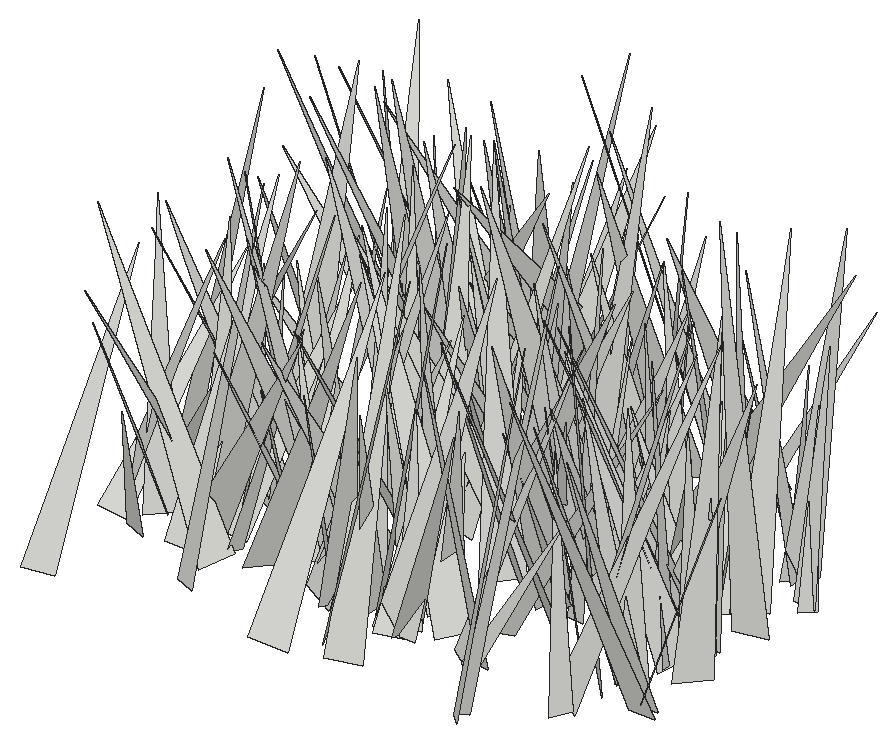
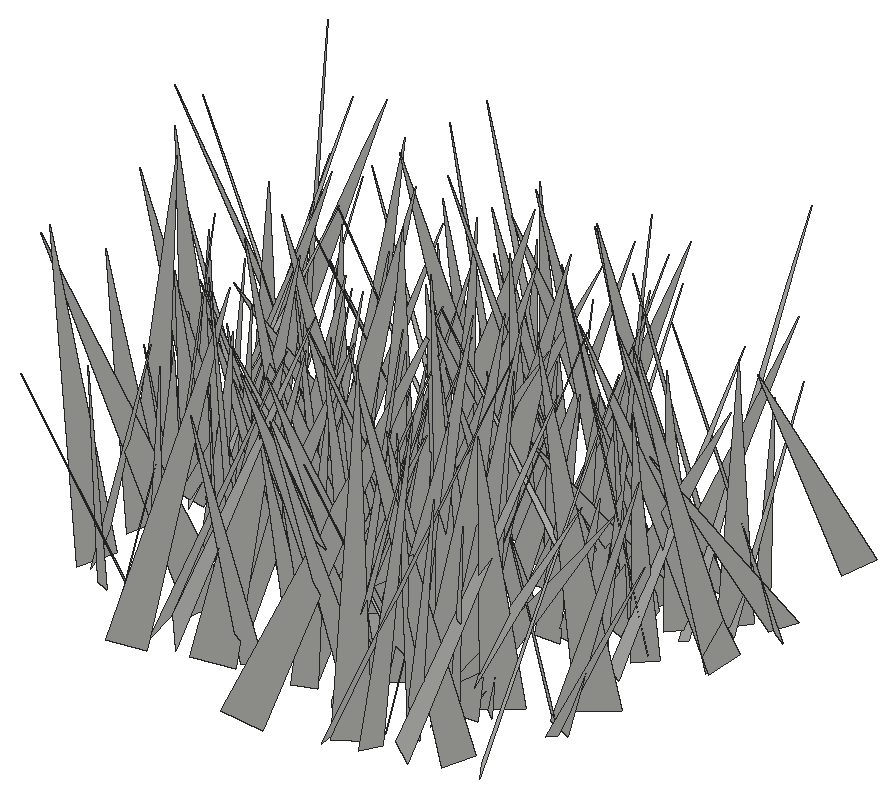
# SketchUp Ruby script. Lengths in inches.
U = 1.inch
M = Sketchup.active_model
def pt(a) = Geom::Point3d.new(a.map { |v| v * U })
def face(e, loops, mat)
  f = e.add_face(loops[0].map { |a| pt(a) })
  loops[1..].each { |l| e.add_face(l.map { |a| pt(a) }).erase! }
  f.material = f.back_material = mat if mat
  f
end
# faces: each face lists its corners as indices into pts; further lists are holes
def faces(e, pts, list, mat = nil) = list.each { |f| face(e, (f[0].is_a?(Array) ? f : [f]).map { |l| l.map { |i| pts[i] } }, mat) }
# xy, xz, yz: faces in a plane at the given z, y or x. An outline is a flat list of corners, or four numbers for a rectangle; further outlines are holes
def ring(l) = l.size == 4 ? [[l[0], l[1]], [l[2], l[1]], [l[2], l[3]], [l[0], l[3]]] : l.each_slice(2).to_a
def flat(e, list, mat, &to3) = list.each { |f| face(e, (f[0].is_a?(Array) ? f : [f]).map { |l| ring(l).map { |u, v| to3.(u, v) } }, mat) }
def xy(e, z, list, mat = nil) = flat(e, list, mat) { |x, y| [x, y, z] }
def xz(e, y, list, mat = nil) = flat(e, list, mat) { |x, z| [x, y, z] }
def yz(e, x, list, mat = nil) = flat(e, list, mat) { |y, z| [x, y, z] }
def lines(e, pts, list) = list.each { |a, b| e.add_line(pt(pts[a]), pt(pts[b])) }
# prism: a flat outline (further loops are holes) pulled along v
def prism(e, loops, v, mat = nil)
  f = face(e, loops, mat); d = Geom::Vector3d.new(v.map { |x| x * U })
  f.pushpull(f.normal.samedirection?(d) ? d.length : -d.length)
end
def box(e, o, s, mat = nil) = prism(e, [[o, [o[0] + s[0], o[1], o[2]], [o[0] + s[0], o[1] + s[1], o[2]], [o[0], o[1] + s[1], o[2]]]], [0, 0, s[2]], mat)
def at(x, y, z, deg = 0) = Geom::Transformation.translation(pt([x, y, z])) * Geom::Transformation.rotation(ORIGIN, Z_AXIS, deg.degrees)
def axes(o, x, y, z) = Geom::Transformation.new([*x, 0, *y, 0, *z, 0, *pt(o).to_a, 1])
def part(name) = M.definitions.add(name)
# library, detail: a bought-in or finely detailed component or shape, given as its bounding box
def library(name, o, s) = part(name).tap { |d| box(d.entities, o, s) }
def detail(e, o, s) = box(e.add_group.entities, o, s)
def put(e, d, t, mat = nil) = e.add_instance(d, t).tap { |i| i.material = mat if mat }
def group(e, t, mat = nil) = e.add_group.tap { |g| g.transformation = t; g.material = mat if mat }.entities
root = M.entities
c1 = part("fur_instance\#9")
p = [[0.8125,0,1.79],[0.67,-0.02,1.48],[0,-0.11,0],[0,0.11,0]]
faces(c1.entities,p,[[0,1,2,3]])
put(root,c1,axes([528.73,42.07,-21.86],[-0.43336,-3.79274,0.22877],[-3.61563,0.48241,1.14868],[1.16807,0.08612,3.64049]))
put(root,c1,axes([527.9,37.6,-21.86],[-4.59878,4.14257,0.47856],[3.69105,4.37512,-2.40275],[1.94062,1.49539,5.70408]))
put(root,c1,axes([538.61,40.67,-21.86],[7.04246,3.4796,1.7186],[3.70112,-7.09298,-0.80545],[-1.16744,-1.49647,7.81378]))
put(root,c1,axes([546.14,38.49,-21.86],[4.5947,4.98178,1.41698],[4.55399,-4.78808,2.06705],[-2.46722,0.43974,6.4542]))
put(root,c1,axes([529.47,45.59,-21.86],[-5.00279,-6.48805,0.18943],[-5.66686,4.48249,3.86684],[3.16501,-2.22958,7.22289]))
put(root,c1,axes([537.7,42.4,-21.86],[5.23742,-3.794,0.7561],[-3.79638,-5.28528,-0.22367],[-0.74406,0.26094,6.46336]))
put(root,c1,axes([537.62,38.52,-21.86],[-1.59566,7.05244,0.57454],[6.94745,1.67322,-1.24356],[1.34162,-0.27674,7.12297]))
put(root,c1,axes([551.11,42.86,-21.86],[-1.75901,-6.72397,0.92553],[-6.70142,1.56883,-1.33876],[-1.07676,1.22044,6.82009]))
put(root,c1,axes([540.875,42.35,-21.86],[5.31861,-1.95589,0.12332],[-1.94358,-5.30997,-0.39374],[-0.25139,-0.32717,5.65315]))
put(root,c1,axes([539,42.79,-21.86],[4.83805,-1.95602,0.87332],[-1.75837,-4.85831,-1.14034],[-1.22345,-0.75248,5.09238]))
put(root,c1,axes([544.34,41.36,-21.86],[2.38056,3.51502,0.37387],[3.33138,-2.08023,-1.65431],[1.18197,-1.21634,3.90969]))
put(root,c1,axes([530.85,43.33,-21.86],[2.77166,-6.45652,0.14972],[-5.9267,-2.47813,2.8503],[2.56578,1.25036,6.42219]))
put(root,c1,axes([548.87,41.07,-21.86],[-4.5869,1.43943,1.05541],[1.33614,4.69877,-0.60151],[1.18347,0.27406,4.76967]))
put(root,c1,axes([537.01,42.99,-21.86],[3.60771,1.96245,2.32029],[2.67745,-3.75626,-0.98607],[-1.43745,-2.07119,3.98679]))
put(root,c1,axes([550.94,43.3125,-21.86],[-0.82643,-5.48525,0.94931],[-5.54864,0.73423,-0.58792],[-0.44918,1.02229,5.51591]))
put(root,c1,axes([532.42,42.1,-21.86],[-6.66331,2.16551,0.21128],[2.17487,6.60915,0.85019],[-0.06344,-0.87375,6.95459]))
put(root,c1,axes([548.43,43.8,-21.86],[-5.2101,-5.93708,2.74108],[-5.84341,5.80017,1.45611],[2.93548,1.00834,7.76362]))
put(root,c1,axes([528.45,44.15,-21.86],[-3.04266,-3.74721,0.50143],[-3.60797,3.07034,1.05183],[1.12942,-0.28668,4.71094]))
put(root,c1,axes([534.29,45.22,-21.86],[-3.9218,-4.42687,0.35438],[-4.07666,3.77609,2.05553],[1.7617,-1.11678,5.54549]))
put(root,c1,axes([540.45,39.26,-21.86],[0.0768,8.17284,0.16546],[8.06568,-0.10268,1.32775],[-1.3295,-0.15078,8.06464]))
put(root,c1,axes([533.91,42.9,-21.86],[6.48225,-3.39085,0.68777],[-3.4557,-6.41712,0.9323],[-0.17042,1.14593,7.25591]))
put(root,c1,axes([544.57,42.02,-21.86],[-3.42492,-4.02626,1.68032],[-4.34426,2.9504,-1.78518],[-0.40205,2.41841,4.97534]))
put(root,c1,axes([540.84,42.4375,-21.86],[-2.37433,3.47563,1.70417],[3.72029,2.6012,-0.12184],[1.06942,-1.33243,4.20745]))
put(root,c1,axes([532.57,40.1,-21.86],[3.83849,6.3713,1.10198],[6.13828,-3.99344,1.70758],[-2.03209,-0.02789,7.23959]))
put(root,c1,axes([536.54,42.74,-21.86],[1.01992,4.1189,1.46608],[4.23417,-0.55549,-1.38501],[1.0893,-1.69737,4.0109]))
put(root,c1,axes([536.79,46.07,-21.86],[-6.04066,-0.63869,2.51357],[0.73038,5.69455,3.20222],[2.48847,-3.22176,5.16172]))
put(root,c1,axes([548.64,44.6,-21.86],[-4.48519,-3.52054,0.94744],[-3.42145,4.58335,0.83384],[1.25916,-0.08621,5.64055]))
put(root,c1,axes([540.61,41.91,-21.86],[-1.59502,6.99566,2.35908],[7.02793,2.17795,-1.70682],[2.26111,-1.83463,6.96922]))
put(root,c1,axes([539.02,43.12,-21.86],[7.03431,3.48518,2.0857],[3.73576,-7.18871,-0.58711],[-1.59396,-1.46769,7.82836]))
put(root,c1,axes([540.55,44.98,-21.86],[-2.23247,-5.83337,0.18602],[-5.6892,2.13065,-1.46288],[-1.30221,0.692,6.07224]))
put(root,c1,axes([546.13,38.92,-21.86],[4.35175,7.0169,0.44581],[6.16578,-4.0605,3.72408],[-3.37917,1.6275,7.36925]))
put(root,c1,axes([541.15,44.47,-21.86],[4.27597,-2.96302,0.67606],[-2.94629,-4.32773,-0.33261],[-0.74558,0.10858,5.19161]))
put(root,c1,axes([534.76,43.93,-21.86],[-2.07432,-2.92088,0.84042],[-3.01146,2.11274,-0.09003],[0.41107,0.73854,3.58137]))
put(root,c1,axes([539.86,44.05,-21.86],[-3.6167,2.28369,2.19841],[2.80718,3.85669,0.61192],[1.47241,-1.74341,4.23336]))
put(root,c1,axes([536.96,44.48,-21.86],[1.50784,-3.41822,0.5063],[-3.4457,-1.52893,-0.06057],[-0.26023,0.4385,3.73552]))
put(root,c1,axes([535.4375,45.76,-21.86],[1.95168,-6.84621,1.26966],[-6.52036,-2.2596,-2.16121],[-2.44285,0.56154,6.78298]))
put(root,c1,axes([536.1875,43.81,-21.86],[4.85202,-3.37562,1.03104],[-3.52041,-4.75453,1.00059],[-0.25408,1.41409,5.82544]))
put(root,c1,axes([548.43,41.87,-21.86],[3.64323,6.95762,0.66244],[6.95502,-3.53547,-1.11744],[0.68929,-1.10109,7.77386]))
put(root,c1,axes([550.3,44.0625,-21.86],[4.88732,1.92922,0.49219],[1.99044,-4.76555,-1.08522],[-0.04774,-1.19066,5.14102]))
put(root,c1,axes([526.9375,43.36,-21.86],[4.20289,4.66758,0.96744],[4.74909,-3.98911,-1.38552],[0.41036,-1.63927,6.12625]))
put(root,c1,axes([542.43,43.31,-21.86],[-4.97351,5.86998,1.15657],[5.9442,4.67754,1.82131],[-0.6788,-2.04794,7.47498]))
put(root,c1,axes([545.41,45.375,-21.86],[-2.96525,-5.05492,0.58848],[-5.08807,2.93137,-0.45808],[-0.10025,0.73898,5.84252]))
put(root,c1,axes([536.84,42.31,-21.86],[3.51205,7.24819,1.1392],[7.33442,-3.43356,-0.76524],[0.20101,-1.35755,8.01781]))
put(root,c1,axes([548.4,42.48,-21.86],[5.62974,5.25868,1.12192],[5.27805,-5.71471,0.30107],[-1.02693,-0.54292,7.69786]))
put(root,c1,axes([536.81,43.6875,-21.86],[-7.94923,-1.56442,0.5472],[-1.62855,7.87073,-1.15603],[0.30767,1.24144,8.0188]))
put(root,c1,axes([549.45,44.27,-21.86],[0.3865,-5.10308,2.42648],[-5.49086,-0.91339,-1.04632],[-1.33405,2.28099,5.00959]))
put(root,c1,axes([543.46,42.06,-21.86],[3.77289,4.9439,0.17652],[4.9129,-3.7705,0.5956],[-0.58026,0.22179,6.19049]))
put(root,c1,axes([531.4,44.71,-21.86],[3.2608,1.42212,0.87051],[1.60342,-3.19897,-0.78016],[-0.45742,-1.07574,3.47082]))
put(root,c1,axes([528.71,43.61,-21.86],[-4.60516,3.74944,1.60687],[3.84875,4.79672,-0.16237],[1.35183,-0.88372,5.93628]))
put(root,c1,axes([532.43,43.15,-21.86],[4.26964,0.47793,1.18834],[0.14194,-4.28676,1.21405],[-1.27296,1.12502,4.1212]))
put(root,c1,axes([530.64,43.48,-21.86],[7.3545,-2.24014,2.18394],[-2.66673,-7.40612,1.38362],[-1.63595,2.00191,7.56257]))
put(root,c1,axes([549.38,44.47,-21.86],[2.70237,-4.42657,2.31196],[-4.83243,-2.98105,-0.05917],[-1.25989,1.93941,5.18593]))
put(root,c1,axes([540.59,41.73,-21.86],[-4.13598,4.27474,0.09369],[4.07434,3.97972,-1.71759],[1.29691,1.13001,5.6947]))
put(root,c1,axes([540.85,44.26,-21.86],[-1.16984,-6.03511,2.92768],[-6.70455,0.96018,-0.69968],[-0.2073,3.00298,6.1075]))
put(root,c1,axes([536.29,44.32,-21.86],[2.31719,-2.3997,1.71249],[-2.74416,-2.55172,0.13746],[-1.07739,1.33819,3.33302]))
put(root,c1,axes([543.58,47.45,-21.86],[6.17469,-3.94346,0.96595],[-3.5616,-6.10514,-2.15707],[-1.94909,-1.33681,7.00177]))
put(root,c1,axes([541.08,44.44,-21.86],[-5.22041,4.31379,0.87725],[4.39805,5.05275,1.32586],[-0.18846,-1.57859,6.64105]))
put(root,c1,axes([535.26,44.52,-21.86],[-3.14224,2.77876,1.0294],[2.91205,3.17344,0.32264],[0.54877,-0.92877,4.18224]))
put(root,c1,axes([530.8,42.125,-21.86],[0.11708,7.08162,0.20269],[7.08451,-0.11681,-0.01106],[0.00771,-0.20285,7.08258]))
put(root,c1,axes([547.01,44.58,-21.86],[-3.71707,-2.68533,1.32909],[-2.9797,3.53518,-1.19076],[0.31439,1.75658,4.42828]))
put(root,c1,axes([538.07,43.82,-21.86],[0.42916,7.00561,1.64499],[7.11073,-0.66598,0.98114],[-1.10544,-1.56418,6.94983]))
put(root,c1,axes([549.8,46.46,-21.86],[-5.95975,2.47486,1.75961],[2.91321,5.75356,1.77469],[0.85695,-2.34763,6.20435]))
put(root,c1,axes([548.92,48.1875,-21.86],[-5.73536,-5.62008,0.65862],[-5.46135,5.74328,1.44982],[1.48081,-0.58562,7.89796]))
put(root,c1,axes([527.3,42.6,-21.86],[-2.44099,4.81015,0.04297],[4.37742,2.2412,-2.21652],[1.99437,0.96814,4.91762]))
put(root,c1,axes([543.95,47.35,-21.86],[-0.76321,-4.71965,0.1503],[-4.6984,0.77422,0.45372],[0.47201,0.07524,4.75939]))
put(root,c1,axes([532.69,47.49,-21.86],[-0.18064,-6.52008,0.8881],[-6.57997,0.17015,-0.08916],[-0.06535,0.89016,6.52198]))
put(root,c1,axes([530,45.06,-21.86],[3.60386,-3.42869,2.87422],[-4.08632,-4.02533,0.32181],[-1.82182,2.24626,4.96388]))
put(root,c1,axes([543.13,48,-21.86],[-0.50575,-5.47671,0.42869],[-5.44927,0.55465,0.65709],[0.69543,0.36321,5.46062]))
put(root,c1,axes([530.62,48.8125,-21.86],[-4.91582,-6.36103,2.07601],[-5.8042,5.33544,2.60426],[3.32923,-0.09063,7.60565]))
put(root,c1,axes([530,46.98,-21.86],[5.79589,4.16761,1.50359],[4.42839,-5.37215,-2.17978],[0.13803,-2.64446,6.79779]))
put(root,c1,axes([529.86,49.0625,-21.86],[-3.98509,-5.15803,0.00595],[-5.07141,3.91953,1.18509],[0.94137,-0.71992,6.40951]))
put(root,c1,axes([543.58,44.37,-21.86],[5.52796,-0.81869,0.7417],[-1.07099,-4.89962,2.57397],[-0.27083,2.66498,4.96017]))
put(root,c1,axes([532.32,46.4,-21.86],[-1.81659,5.58818,1.87966],[5.39696,0.78429,2.88421],[-2.37355,-2.49359,5.11948]))
put(root,c1,axes([550.4375,46.52,-21.86],[-3.98978,2.11987,2.03955],[2.3526,4.36264,0.06771],[1.76604,-1.02247,4.51748]))
put(root,c1,axes([531.44,46.29,-21.86],[1.95895,3.98258,1.69888],[4.26762,-2.09086,-0.01944],[-0.73116,-1.53362,4.43825]))
put(root,c1,axes([527.26,46.05,-21.86],[6.85637,-0.90607,0.05149],[-0.90407,-6.7849,0.99057],[0.07926,0.98874,6.84468]))
put(root,c1,axes([541.9375,47.53,-21.86],[-2.91722,-4.26379,0.81225],[-4.33997,2.88016,-0.46811],[0.06569,0.93518,5.14499]))
put(root,c1,axes([551.03,45.86,-21.86],[5.64429,-3.09602,3.33103],[-3.78051,-6.14532,0.69416],[-2.52761,2.27789,6.40012]))
put(root,c1,axes([550.2,47.54,-21.86],[2.54214,-2.62214,0.84113],[-2.70032,-2.59808,0.06187],[-0.53981,0.64801,3.65161]))
put(root,c1,axes([531.66,43.93,-21.86],[-3.68567,4.23937,0.30212],[3.60627,3.33103,-2.74713],[2.24908,1.60613,4.89997]))
put(root,c1,axes([549.65,48.41,-21.86],[-5.40162,-4.18627,0.13743],[-4.18531,5.38577,-0.4449],[-0.16419,0.43574,6.81941]))
put(root,c1,axes([544.92,48.96,-21.86],[2.25117,-4.50739,0.41367],[-4.42833,-2.28883,-0.84056],[-0.93676,-0.01195,4.96767]))
put(root,c1,axes([529.57,47.63,-21.86],[-2.45808,3.26284,2.53045],[3.74921,2.99751,-0.22312],[1.72995,-1.86016,4.07903]))
put(root,c1,axes([549.67,46.23,-21.86],[-5.30333,-1.20318,1.41609],[-1.56427,5.2022,-1.4382],[1.00301,1.75149,5.24448]))
put(root,c1,axes([533.125,45.6,-21.86],[-2.87102,4.68172,0.40163],[4.57171,2.89185,-1.02921],[1.08596,0.20316,5.39463]))
put(root,c1,axes([534.57,47.97,-21.86],[1.52627,-4.48364,1.33128],[-4.39877,-0.90019,2.01128],[1.58937,1.81423,4.28804]))
put(root,c1,axes([548.07,48.19,-21.86],[3.29636,-5.4576,1.30622],[-5.51274,-2.86598,1.93739],[1.04942,2.08768,6.07437]))
put(root,c1,axes([533.3,48.54,-21.86],[0.46643,-4.66615,1.44002],[-4.86096,-0.58186,-0.31092],[-0.46655,1.39737,4.67909]))
put(root,c1,axes([527.69,45.84,-21.86],[-6.79191,0.51616,3.38033],[-0.49773,7.28774,-2.11287],[3.3831,2.10844,6.47551]))
put(root,c1,axes([536.42,49.17,-21.86],[4.0303,-5.81988,3.12764],[-5.66664,-4.92868,-1.86917],[-3.39741,1.31665,6.82792]))
put(root,c1,axes([550.01,47.5625,-21.86],[-2.87037,3.7349,1.34525],[3.80013,3.06525,-0.40189],[1.14815,-0.80807,4.69329]))
put(root,c1,axes([541.7,49.74,-21.86],[4.03439,-1.67825,0.01541],[-1.64329,-3.95818,-0.85174],[-0.3411,-0.78061,4.28572]))
put(root,c1,axes([546.64,50,-21.86],[4.66467,-0.77947,0.02704],[-0.7406,-4.47818,-1.32848],[-0.24456,-1.30606,4.53893]))
put(root,c1,axes([541.22,47.35,-21.86],[-6.71454,4.39928,1.56364],[4.39375,6.8803,-0.4901],[1.57912,-0.43767,8.0124]))
put(root,c1,axes([546.6,48.36,-21.86],[0.69151,3.97199,1.28395],[4.17346,-0.6309,-0.296],[0.08642,-1.31479,4.02085]))
put(root,c1,axes([549.42,48.54,-21.86],[-1.85647,3.95367,0.8299],[3.82368,1.42492,1.76516],[-1.30372,-1.4508,3.99527]))
put(root,c1,axes([545,46.75,-21.86],[2.80201,6.02167,1.40008],[5.6342,-3.12002,2.14317],[-2.54489,-0.27744,6.28638]))
put(root,c1,axes([539.17,50.17,-21.86],[3.33833,-6.51025,0.54896],[-6.14625,-2.92038,2.74304],[2.21549,1.70799,6.78259]))
put(root,c1,axes([544.76,47.95,-21.86],[2.02103,5.13059,0.73898],[5.12624,-1.86067,-1.10143],[0.76856,-1.08099,5.40318]))
put(root,c1,axes([539.75,50.08,-21.86],[-4.43221,4.72995,1.58971],[4.78005,3.41433,3.16821],[-1.43205,-3.24253,5.65503]))
put(root,c1,axes([550.18,48.18,-21.86],[1.43677,3.63281,1.03111],[3.57622,-1.66329,0.8769],[-1.21291,-0.60083,3.80693]))
put(root,c1,axes([543.33,49.38,-21.86],[-5.71627,0.02456,1.51927],[0.09668,5.9079,0.26822],[1.51639,-0.28405,5.71003]))
put(root,c1,axes([532.5625,48.18,-21.86],[-1.14245,4.14217,0.46464],[4.01441,0.96381,1.27839],[-1.12161,-0.76952,4.10226]))
put(root,c1,axes([532.27,46.87,-21.86],[5.64336,5.1887,0.30355],[5.15395,-5.64438,0.66329],[-0.67191,0.28398,7.63742]))
put(root,c1,axes([540.6,50.17,-21.86],[-1.63509,-3.83691,0.93062],[-3.94815,1.58786,-0.39017],[-0.00453,1.00909,4.15248]))
put(root,c1,axes([537.7,51.52,-21.86],[-0.82646,-4.24361,0.01629],[-4.06802,0.79698,1.2278],[1.20816,-0.21938,4.14533]))
put(root,c1,axes([540.83,48.28,-21.86],[-4.40287,4.25609,0.42122],[4.26988,4.40886,0.08361],[0.24458,-0.35298,6.12311]))
put(root,c1,axes([541.32,52.15,-21.86],[5.28612,-6.00356,2.19792],[-5.60526,-5.72373,-2.15328],[-3.07484,0.113,7.70384]))
put(root,c1,axes([538.91,52.64,-21.86],[-4.92711,-3.11526,0.5387],[-2.69685,4.66208,2.29422],[1.64986,-1.68274,5.3589]))
put(root,c1,axes([540.53,48.1,-21.86],[-4.43133,1.84787,0.51045],[1.62369,4.30117,-1.47494],[1.01922,1.18203,4.56901]))
put(root,c1,axes([546.48,50.24,-21.86],[-2.57629,-2.49445,0.93197],[-2.62206,2.60252,-0.28257],[0.46438,0.85602,3.57488]))
put(root,c1,axes([537.45,48.54,-21.86],[-2.63415,6.93544,1.64719],[7.09873,2.71215,-0.06728],[0.64926,-1.51533,7.41852]))
put(root,c1,axes([546.39,49.64,-21.86],[-5.10853,0.04095,1.59169],[-0.11644,5.32521,-0.51071],[1.58796,0.52222,5.08311]))
put(root,c1,axes([550.53,49.77,-21.86],[-0.94907,-6.99906,3.73248],[-7.88487,0.42284,-1.21201],[-0.8643,3.82797,6.95835]))
put(root,c1,axes([539.19,50.53,-21.86],[-4.76846,2.17787,1.48985],[2.383,4.8757,0.4998],[1.13316,-1.08876,5.21838]))
put(root,c1,axes([541.77,49.44,-21.86],[-6.70794,-1.60484,0.19836],[-1.59675,6.44001,-1.8942],[-0.25542,1.88735,6.63204]))
put(root,c1,axes([529.42,50.46,-21.86],[1.77196,3.84512,1.4323],[4.08534,-1.50774,-1.0065],[0.38272,-1.70823,4.11239]))
put(root,c1,axes([538.5,51.03,-21.86],[0.92533,-3.44435,1.34936],[-3.58141,-1.18238,-0.56215],[-0.92618,1.13092,3.52189]))
put(root,c1,axes([535.49,49.16,-21.86],[-0.40472,6.25604,0.83945],[6.18781,0.22712,1.29072],[-1.24649,-0.90382,6.13481]))
put(root,c1,axes([537.27,49.92,-21.86],[3.77133,0.16267,0.95437],[-0.10228,-3.74984,1.04331],[-0.96272,1.03561,3.6278]))
put(root,c1,axes([536.12,53.39,-21.86],[4.85347,-3.26157,0.26621],[-3.0891,-4.72355,-1.55255],[-1.07988,-1.1468,5.6377]))
put(root,c1,axes([543.64,49.34,-21.86],[1.45734,4.18221,0.34787],[4.02467,-1.49715,1.13854],[-1.18907,0.05834,4.28]))
put(root,c1,axes([539.02,50.97,-21.86],[4.06657,-2.17936,1.39694],[-2.40276,-4.14574,0.52683],[-0.9632,1.14071,4.58356]))
put(root,c1,axes([547.73,52.09,-21.86],[-5.52938,-3.456,2.07939],[-3.45701,5.87854,0.57763],[2.07771,0.58365,6.49494]))
put(root,c1,axes([548.52,50.49,-21.86],[3.3556,2.16226,1.21696],[2.08771,-3.56664,0.58052],[-1.34083,-0.14202,3.94948]))
put(root,c1,axes([538.58,51.82,-21.86],[2.73482,-5.11249,1.4467],[-5.08402,-2.04521,2.38319],[1.54377,2.32148,5.28557]))
put(root,c1,axes([548.99,50.5,-21.86],[-1.86757,4.60063,0.33127],[4.58089,1.80817,0.71369],[-0.53944,-0.57279,4.91369]))
put(root,c1,axes([537.76,49.16,-21.86],[2.14003,7.20036,0.0672],[7.19519,-2.14104,0.27303],[-0.28086,0.01341,7.50668]))
put(root,c1,axes([528.625,51.48,-21.86],[-2.68799,6.56885,2.98447],[6.8694,3.30396,-1.08507],[2.20641,-2.2839,7.01411]))
put(root,c1,axes([541.61,52.01,-21.86],[-0.77235,4.89048,2.70767],[4.92537,1.88806,-2.00519],[2.64368,-2.08884,4.52687]))
put(root,c1,axes([528.9375,53.3,-21.86],[-1.73362,-4.79917,0.85478],[-4.86621,1.65027,-0.60395],[-0.28757,1.00633,5.06683]))
put(root,c1,axes([533.86,53.22,-21.86],[7.52805,-0.18805,1.99939],[0.07054,-7.72753,-0.99239],[-2.00698,-0.97696,7.46472]))
put(root,c1,axes([528.79,53.91,-21.86],[-3.56897,-0.50146,0.42511],[-0.28446,3.29362,1.49696],[0.59267,-1.43888,3.27843]))
put(root,c1,axes([535.26,54.02,-21.86],[-6.0404,2.2493,3.21945],[3.13358,6.3206,1.46334],[2.36747,-2.62704,6.2773]))
put(root,c1,axes([546.09,51.66,-21.86],[-5.59826,1.4556,0.99849],[1.35798,5.67289,-0.65612],[1.12768,0.39476,5.74707]))
put(root,c1,axes([539.2,53.61,-21.86],[-0.83843,-4.56243,0.7415],[-4.45874,0.59959,-1.35228],[-1.2187,0.94513,4.43735]))
put(root,c1,axes([536.75,51.11,-21.86],[-3.134,4.47853,0.59876],[4.43295,3.18866,-0.64743],[0.8745,-0.1137,5.42771]))
put(root,c1,axes([539.98,52.18,-21.86],[1.92341,3.31368,0.82854],[3.39872,-1.95136,-0.08567],[-0.34002,-0.7604,3.83049]))
put(root,c1,axes([549.52,50.99,-21.86],[-5.92088,3.75972,1.43779],[3.50525,6.07307,-1.44586],[1.97886,0.49178,6.86307]))
put(root,c1,axes([542.92,54.02,-21.86],[-1.01411,-6.0227,1.51425],[-5.97973,0.53295,-1.88497],[-1.67593,1.7428,5.80932]))
put(root,c1,axes([532.57,55.91,-21.66],[-6.5639,-4.29471,0.69968],[-4.06333,6.50273,1.7952],[1.55674,-1.13527,7.63588]))
put(root,c1,axes([541.65,51.49,-21.86],[1.82525,7.99707,1.79582],[8.16577,-1.93273,0.30716],[-0.70587,-1.67961,8.19697]))
put(root,c1,axes([532.4,54.77,-21.86],[1.08245,-7.41016,1.80762],[-7.58562,-1.23679,-0.52762],[-0.7977,1.70574,7.47019]))
put(root,c1,axes([550.6875,52.61,-21.86],[0.70725,4.81258,1.31899],[4.97344,-0.78845,0.21001],[-0.40688,-1.27212,4.85974]))
put(root,c1,axes([551.09,52.32,-21.86],[-3.45785,1.40655,0.59459],[1.25916,3.45892,-0.85969],[0.86397,0.58836,3.63264]))
put(root,c1,axes([533.38,54.75,-21.86],[1.42395,-7.42701,2.10024],[-7.62151,-1.69014,-0.80943],[-1.21824,1.89264,7.51884]))
put(root,c1,axes([542.98,54.21,-21.86],[4.1746,-2.61988,2.8232],[-2.37692,-5.02847,-1.15163],[-3.03059,0.33503,4.79215]))
put(root,c1,axes([538.32,55.97,-21.86],[3.38656,-3.48151,1.0277],[-2.77448,-3.38882,-2.33752],[-2.3408,-1.02022,4.25743]))
put(root,c1,axes([540.75,52.47,-21.86],[5.15508,0.33774,1.32609],[0.02228,-5.18864,1.23487],[-1.36825,1.188,5.01637]))
put(root,c1,axes([531.95,53.66,-21.86],[-4.37552,-5.12362,2.64469],[-5.63456,4.50416,-0.59611],[1.22377,2.41912,6.71129]))
put(root,c1,axes([537.37,54.56,-21.86],[-6.26815,-2.22604,2.13273],[-2.17784,6.6177,0.5065],[2.18193,0.21043,6.63238]))
put(root,c1,axes([532.93,54.44,-21.86],[-3.83855,4.56526,0.77541],[4.17711,2.97899,3.13921],[-1.99865,-2.54191,5.07163]))
put(root,c1,axes([529.47,52.95,-21.86],[2.58432,3.47984,0.90101],[3.42396,-2.72089,0.68775],[-1.09434,-0.29537,4.2796]))
put(root,c1,axes([537.5625,52.39,-21.86],[6.4283,2.09347,0.22673],[2.03253,-6.35917,1.08941],[-0.55031,0.96716,6.67224]))
put(root,c1,axes([541.04,52.05,-21.86],[-5.03448,1.97141,0.87824],[1.57247,4.87743,-1.93439],[1.47821,1.52579,5.04882]))
put(root,c1,axes([542.91,53.96,-21.86],[5.91365,2.78735,2.33328],[2.94924,-6.28377,0.03183],[-2.12497,-0.96423,6.53755]))
put(root,c1,axes([537.25,54.18,-21.86],[5.91491,-0.67607,1.90084],[-0.77835,-6.19702,0.21795],[-1.8613,0.44302,5.94943]))
put(root,c1,axes([544.11,54.25,-21.86],[6.07863,-4.42165,0.21276],[-4.21796,-5.67554,2.55792],[1.3435,2.18706,7.06807]))
put(root,c1,axes([549.4,53.89,-21.86],[-5.62081,-1.07857,0.79033],[-1.22962,5.511,-1.22409],[0.52534,1.35906,5.59093]))
put(root,c1,axes([541.27,52.9,-21.86],[-5.01986,0.40192,1.5189],[-0.17545,4.90978,-1.87904],[1.56135,1.84392,4.67223]))
put(root,c1,axes([549.375,54.01,-21.86],[-5.57842,3.33095,2.99608],[3.28064,6.29556,-0.89096],[3.05108,-0.67911,6.43585]))
put(root,c1,axes([537.89,56.59,-21.86],[0.34868,-5.31048,0.36463],[-5.26358,-0.28954,0.81646],[0.79301,0.41316,5.25892]))
put(root,c1,axes([529.1875,57.45,-21.86],[-6.21102,-4.85766,0.88936],[-4.64444,6.23147,1.60082],[1.67841,-0.73247,7.72082]))
put(root,c1,axes([541.51,57.27,-21.86],[2.6009,-7.25193,0.96085],[-7.2129,-2.71231,-0.94648],[-1.21974,0.57558,7.64587]))
put(root,c1,axes([541.98,56.17,-21.86],[4.17117,1.8451,1.43695],[2.27213,-3.89306,-1.59669],[-0.55375,-2.07548,4.27243]))
put(root,c1,axes([548.04,55.36,-21.86],[-1.72893,-3.46771,1.76985],[-3.62718,2.13831,0.64633],[1.41454,1.24466,3.82053]))
put(root,c1,axes([533.16,53.71,-21.86],[-6.11447,-3.98639,0.59028],[-3.68819,5.10346,-3.73879],[-1.62389,3.41906,6.26894]))
put(root,c1,axes([535.8,53.94,-21.86],[-4.22823,5.63878,0.60494],[5.64653,4.11564,1.10357],[-0.52773,-1.14251,6.96102]))
put(root,c1,axes([537.85,60.19,-21.66],[5.96387,-5.74764,0.45925],[-4.68382,-5.21453,-4.43673],[-3.36276,-2.93042,6.99418]))
put(root,c1,axes([536.2,57.1,-21.86],[-4.57132,-4.01454,0.83204],[-3.89365,4.6413,1.00178],[1.28384,-0.21818,6.00082]))
put(root,c1,axes([530.22,57.43,-21.86],[1.13503,-7.67663,0.6742],[-6.50823,-0.58999,4.2389],[4.12651,1.18099,6.50005]))
put(root,c1,axes([544.69,58.2,-21.86],[3.73251,-5.71066,0.85994],[-5.41751,-3.81707,-1.83396],[-2.00044,-0.31799,6.57114]))
put(root,c1,axes([531.4,53.43,-21.86],[-4.20767,6.2047,0.57896],[6.20765,4.23458,-0.26697],[0.54635,-0.32858,7.49209]))
put(root,c1,axes([536.37,52.91,-21.86],[3.4696,4.95294,0.18512],[4.68916,-3.35343,1.83583],[-1.60551,0.90933,5.7619]))
put(root,c1,axes([533.15,56.24,-21.86],[5.21956,1.10973,1.69595],[1.36173,-5.39042,-0.66376],[-1.50115,-1.03121,5.29478]))
put(root,c1,axes([546.17,54.77,-21.86],[-5.50715,-0.70612,1.61288],[-1.08889,5.52799,-1.29784],[1.38358,1.53996,5.39842]))
put(root,c1,axes([532.21,58.17,-21.86],[-4.57477,-6.03245,0.25242],[-6.03633,4.57654,-0.02819],[0.13005,0.21817,7.57088]))
put(root,c1,axes([534.64,59.38,-21.66],[-6.99156,-3.62516,0.34789],[-3.32905,6.6672,2.57109],[1.47657,-2.13338,7.444]))
put(root,c1,axes([538.11,52.27,-21.86],[7.29611,1.84526,3.54482],[-0.04664,-7.33917,3.91643],[-3.99607,3.45479,6.4265]))
put(root,c1,axes([532.01,55.42,-21.66],[2.11114,4.26728,1.69749],[4.08085,-2.60007,1.46097],[-2.10662,-0.76029,4.53125]))
put(root,c1,axes([544.53,56.48,-21.86],[-7.29173,-1.24054,0.1592],[-1.24954,7.26646,-0.60898],[0.05425,0.6271,7.37139]))
put(root,c1,axes([536.59,54.78,-21.86],[-2.83058,6.09964,1.95872],[5.76034,3.3604,-2.14023],[2.80369,-0.74599,6.37473]))
put(root,c1,axes([543.72,56.67,-21.66],[-6.31099,-5.2237,1.0112],[-5.28027,5.95593,-2.18722],[-0.65451,2.31907,7.89505]))
put(root,c1,axes([534.15,58.61,-21.86],[2.97455,-6.14482,0.55918],[-6.16848,-2.94679,0.43089],[0.14598,0.69067,6.8133]))
put(root,c1,axes([532.79,56.8,-21.86],[1.70203,4.17643,2.24286],[4.55719,-2.09788,0.44817],[-1.30578,-1.87783,4.48761]))
put(root,c1,axes([536.02,55.89,-21.86],[0.03547,5.69131,1.501],[5.73382,0.30561,-1.29426],[1.32938,-1.46999,5.5423]))
put(root,c1,axes([536.53,56.11,-21.86],[-6.24639,-1.28271,0.8155],[-1.43317,6.11916,-1.35263],[0.50635,1.49608,6.23162]))
put(root,c1,axes([533.27,58.58,-21.86],[5.81845,-0.62274,2.18855],[-0.03101,-6.03017,-1.6334],[-2.27522,-1.51035,5.61909]))
put(root,c1,axes([540.27,56.54,-21.86],[0.29151,4.89673,1.62599],[5.06271,0.04273,-1.03633],[0.99541,-1.65136,4.79468]))
put(root,c1,axes([545.93,57.31,-21.86],[-3.07283,-1.79032,0.75021],[-1.87261,3.10397,-0.26279],[0.51124,0.60869,3.54662]))
put(root,c1,axes([545.05,56.57,-21.86],[3.55975,3.91646,0.08522],[3.79537,-3.41954,-1.38552],[0.97011,-0.99289,5.10792]))
put(root,c1,axes([533.8,56.96,-21.86],[-3.37291,-1.64413,0.77782],[-1.79286,3.28135,-0.83849],[0.30629,1.10194,3.65741]))
